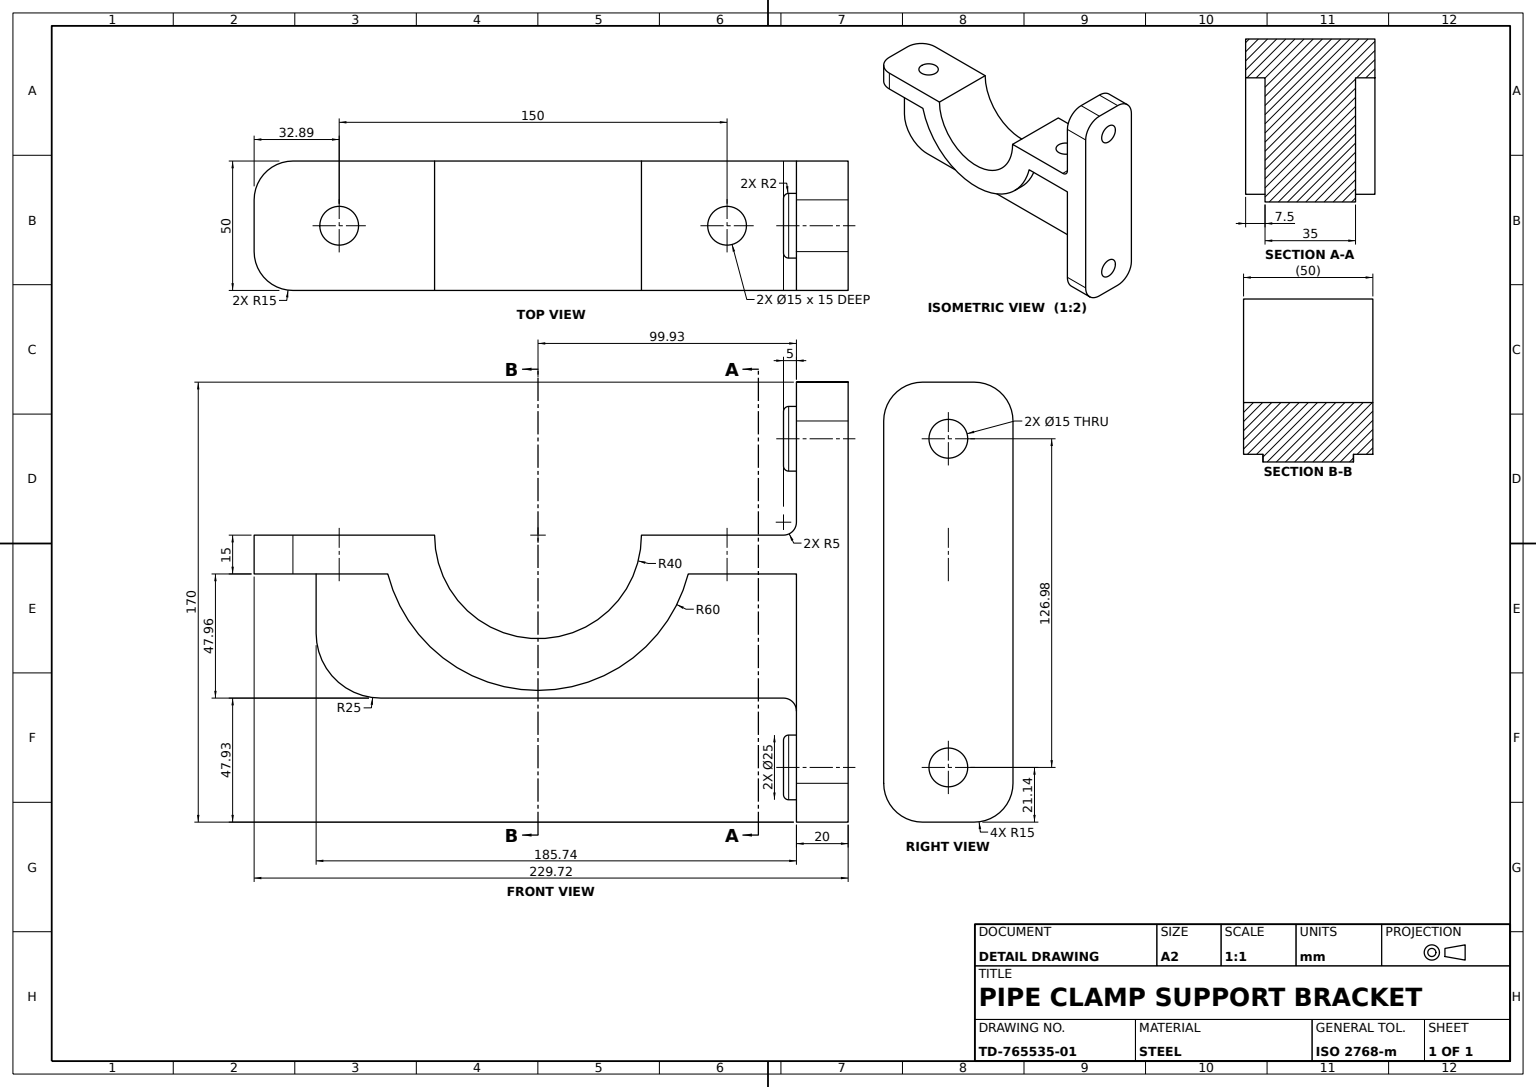
ISO-10303-21;
HEADER;
FILE_DESCRIPTION((''),'2;1');
FILE_NAME('','',(''),(''),'','','');
FILE_SCHEMA(('AUTOMOTIVE_DESIGN'));
ENDSEC;
DATA;
#1=APPLICATION_CONTEXT('');
#2=PRODUCT_CONTEXT('',#1,'mechanical');
#3=PRODUCT('','','',(#2));
#4=PRODUCT_DEFINITION_FORMATION('','',#3);
#5=PRODUCT_DEFINITION_CONTEXT('',#1,'design');
#6=PRODUCT_DEFINITION('','',#4,#5);
#7=PRODUCT_DEFINITION_SHAPE('','',#6);
#8=(LENGTH_UNIT()NAMED_UNIT(*)SI_UNIT(.MILLI.,.METRE.));
#9=(NAMED_UNIT(*)PLANE_ANGLE_UNIT()SI_UNIT($,.RADIAN.));
#10=(NAMED_UNIT(*)SI_UNIT($,.STERADIAN.)SOLID_ANGLE_UNIT());
#11=UNCERTAINTY_MEASURE_WITH_UNIT(LENGTH_MEASURE(1.E-05),#8,'distance_accuracy_value','');
#12=(GEOMETRIC_REPRESENTATION_CONTEXT(3)GLOBAL_UNCERTAINTY_ASSIGNED_CONTEXT((#11))GLOBAL_UNIT_ASSIGNED_CONTEXT((#8,#9,#10))REPRESENTATION_CONTEXT('',''));
#13=CARTESIAN_POINT('',(-17.5,10.889968,205.743047));
#14=VERTEX_POINT('',#13);
#15=CARTESIAN_POINT('',(-17.5,-12.074588,205.743047));
#16=VERTEX_POINT('',#15);
#17=DIRECTION('',(0.,-1.,0.));
#18=VECTOR('',#17,1000.);
#19=LINE('',#13,#18);
#20=EDGE_CURVE('',#14,#16,#19,.T.);
#21=ORIENTED_EDGE('',*,*,#20,.F.);
#22=CARTESIAN_POINT('',(-17.5,10.889968,178.029229));
#23=VERTEX_POINT('',#22);
#24=DIRECTION('',(0.,0.,1.));
#25=VECTOR('',#24,1000.);
#26=LINE('',#22,#25);
#27=EDGE_CURVE('',#23,#14,#26,.T.);
#28=ORIENTED_EDGE('',*,*,#27,.F.);
#29=CARTESIAN_POINT('',(-17.5,10.889968,61.839729));
#30=VERTEX_POINT('',#29);
#31=CARTESIAN_POINT('',(-17.5,25.889968,119.934479));
#32=DIRECTION('',(-1.,0.,0.));
#33=DIRECTION('',(0.,0.,-1.));
#34=AXIS2_PLACEMENT_3D('',#31,#32,#33);
#35=CIRCLE('',#34,60.);
#36=EDGE_CURVE('',#30,#23,#35,.T.);
#37=ORIENTED_EDGE('',*,*,#36,.F.);
#38=CARTESIAN_POINT('',(-17.5,10.889968,20.));
#39=VERTEX_POINT('',#38);
#40=LINE('',#29,#25);
#41=EDGE_CURVE('',#39,#30,#40,.T.);
#42=ORIENTED_EDGE('',*,*,#41,.F.);
#43=CARTESIAN_POINT('',(-17.5,-42.074588,20.));
#44=VERTEX_POINT('',#43);
#45=DIRECTION('',(0.,1.,0.));
#46=VECTOR('',#45,1000.);
#47=LINE('',#38,#46);
#48=EDGE_CURVE('',#44,#39,#47,.T.);
#49=ORIENTED_EDGE('',*,*,#48,.F.);
#50=CARTESIAN_POINT('',(-17.5,-37.074588,25.));
#51=VERTEX_POINT('',#50);
#52=CARTESIAN_POINT('',(-17.5,-42.074588,25.));
#53=DIRECTION('',(1.,0.,0.));
#54=AXIS2_PLACEMENT_3D('',#52,#53,#33);
#55=CIRCLE('',#54,5.);
#56=EDGE_CURVE('',#44,#51,#55,.T.);
#57=ORIENTED_EDGE('',*,*,#56,.T.);
#58=CARTESIAN_POINT('',(-17.5,-37.074588,180.743047));
#59=VERTEX_POINT('',#58);
#60=CARTESIAN_POINT('',(-17.5,-37.074588,205.743047));
#61=VECTOR('',#33,1000.);
#62=LINE('',#60,#61);
#63=EDGE_CURVE('',#59,#51,#62,.T.);
#64=ORIENTED_EDGE('',*,*,#63,.F.);
#65=CARTESIAN_POINT('',(-17.5,-12.074588,180.743047));
#66=AXIS2_PLACEMENT_3D('',#65,#32,#33);
#67=CIRCLE('',#66,25.);
#68=EDGE_CURVE('',#59,#16,#67,.T.);
#69=ORIENTED_EDGE('',*,*,#68,.T.);
#70=EDGE_LOOP('',(#21,#28,#37,#42,#49,#57,#64,#69));
#71=FACE_OUTER_BOUND('',#70,.T.);
#72=AXIS2_PLACEMENT_3D('',#31,#53,#33);
#73=PLANE('',#72);
#74=ADVANCED_FACE('',(#71),#73,.F.);
#75=CARTESIAN_POINT('',(25.,25.889968,79.934479));
#76=VERTEX_POINT('',#75);
#77=CARTESIAN_POINT('',(-25.,25.889968,79.934479));
#78=VERTEX_POINT('',#77);
#79=VECTOR('',#32,1000.);
#80=LINE('',#75,#79);
#81=EDGE_CURVE('',#76,#78,#80,.T.);
#82=ORIENTED_EDGE('',*,*,#81,.F.);
#83=CARTESIAN_POINT('',(25.,25.889968,25.));
#84=VERTEX_POINT('',#83);
#85=LINE('',#75,#61);
#86=EDGE_CURVE('',#76,#84,#85,.T.);
#87=ORIENTED_EDGE('',*,*,#86,.T.);
#88=CARTESIAN_POINT('',(-25.,25.889968,25.));
#89=VERTEX_POINT('',#88);
#90=LINE('',#88,#79);
#91=EDGE_CURVE('',#84,#89,#90,.T.);
#92=ORIENTED_EDGE('',*,*,#91,.T.);
#93=LINE('',#77,#61);
#94=EDGE_CURVE('',#78,#89,#93,.T.);
#95=ORIENTED_EDGE('',*,*,#94,.F.);
#96=EDGE_LOOP('',(#82,#87,#92,#95));
#97=FACE_OUTER_BOUND('',#96,.T.);
#98=CARTESIAN_POINT('',(0.,25.889968,54.322731));
#99=VERTEX_POINT('',#98);
#100=CARTESIAN_POINT('',(0.,25.889968,39.322731));
#101=VERTEX_POINT('',#100);
#102=CARTESIAN_POINT('',(0.,25.889968,46.822731));
#103=AXIS2_PLACEMENT_3D('',#102,#45,#24);
#104=CIRCLE('',#103,7.5);
#105=EDGE_CURVE('',#99,#101,#104,.T.);
#106=ORIENTED_EDGE('',*,*,#105,.F.);
#107=EDGE_CURVE('',#101,#99,#104,.T.);
#108=ORIENTED_EDGE('',*,*,#107,.F.);
#109=EDGE_LOOP('',(#106,#108));
#110=FACE_BOUND('',#109,.T.);
#111=AXIS2_PLACEMENT_3D('',#75,#45,#24);
#112=PLANE('',#111);
#113=ADVANCED_FACE('',(#97,#110),#112,.T.);
#114=CARTESIAN_POINT('',(10.,25.889968,229.717626));
#115=VERTEX_POINT('',#114);
#116=CARTESIAN_POINT('',(25.,25.889968,214.717626));
#117=VERTEX_POINT('',#116);
#118=CARTESIAN_POINT('',(10.,25.889968,214.717626));
#119=AXIS2_PLACEMENT_3D('',#118,#45,#33);
#120=CIRCLE('',#119,15.);
#121=EDGE_CURVE('',#115,#117,#120,.T.);
#122=ORIENTED_EDGE('',*,*,#121,.F.);
#123=CARTESIAN_POINT('',(10.,10.889968,229.717626));
#124=VERTEX_POINT('',#123);
#125=LINE('',#114,#46);
#126=EDGE_CURVE('',#124,#115,#125,.T.);
#127=ORIENTED_EDGE('',*,*,#126,.F.);
#128=CARTESIAN_POINT('',(25.,10.889968,214.717626));
#129=VERTEX_POINT('',#128);
#130=CARTESIAN_POINT('',(10.,10.889968,214.717626));
#131=AXIS2_PLACEMENT_3D('',#130,#17,#33);
#132=CIRCLE('',#131,15.);
#133=EDGE_CURVE('',#129,#124,#132,.T.);
#134=ORIENTED_EDGE('',*,*,#133,.F.);
#135=LINE('',#128,#18);
#136=EDGE_CURVE('',#117,#129,#135,.T.);
#137=ORIENTED_EDGE('',*,*,#136,.F.);
#138=EDGE_LOOP('',(#122,#127,#134,#137));
#139=FACE_OUTER_BOUND('',#138,.T.);
#140=AXIS2_PLACEMENT_3D('',#130,#17,#53);
#141=CYLINDRICAL_SURFACE('',#140,15.);
#142=ADVANCED_FACE('',(#139),#141,.T.);
#143=CARTESIAN_POINT('',(7.5,-63.86192,25.));
#144=VERTEX_POINT('',#143);
#145=CARTESIAN_POINT('',(-7.5,-63.86192,25.));
#146=VERTEX_POINT('',#145);
#147=CARTESIAN_POINT('',(0.,-63.86192,25.));
#148=AXIS2_PLACEMENT_3D('',#147,#24,#53);
#149=CIRCLE('',#148,7.5);
#150=EDGE_CURVE('',#144,#146,#149,.T.);
#151=ORIENTED_EDGE('',*,*,#150,.T.);
#152=CARTESIAN_POINT('',(-7.5,-63.86192,0.));
#153=VERTEX_POINT('',#152);
#154=CARTESIAN_POINT('',(-7.5,-63.86192,-5.));
#155=LINE('',#154,#25);
#156=EDGE_CURVE('',#153,#146,#155,.T.);
#157=ORIENTED_EDGE('',*,*,#156,.F.);
#158=CARTESIAN_POINT('',(7.5,-63.86192,0.));
#159=VERTEX_POINT('',#158);
#160=CARTESIAN_POINT('',(0.,-63.86192,0.));
#161=AXIS2_PLACEMENT_3D('',#160,#24,#53);
#162=CIRCLE('',#161,7.5);
#163=EDGE_CURVE('',#159,#153,#162,.T.);
#164=ORIENTED_EDGE('',*,*,#163,.F.);
#165=CARTESIAN_POINT('',(7.5,-63.86192,-5.));
#166=LINE('',#165,#25);
#167=EDGE_CURVE('',#159,#144,#166,.T.);
#168=ORIENTED_EDGE('',*,*,#167,.T.);
#169=EDGE_LOOP('',(#151,#157,#164,#168));
#170=FACE_OUTER_BOUND('',#169,.T.);
#171=CARTESIAN_POINT('',(0.,-63.86192,-5.));
#172=AXIS2_PLACEMENT_3D('',#171,#24,#53);
#173=CYLINDRICAL_SURFACE('',#172,7.5);
#174=ADVANCED_FACE('',(#170),#173,.F.);
#175=CARTESIAN_POINT('',(7.5,63.122207,0.));
#176=VERTEX_POINT('',#175);
#177=CARTESIAN_POINT('',(-7.5,63.122207,0.));
#178=VERTEX_POINT('',#177);
#179=CARTESIAN_POINT('',(0.,63.122207,0.));
#180=AXIS2_PLACEMENT_3D('',#179,#24,#53);
#181=CIRCLE('',#180,7.5);
#182=EDGE_CURVE('',#176,#178,#181,.T.);
#183=ORIENTED_EDGE('',*,*,#182,.T.);
#184=EDGE_CURVE('',#178,#176,#181,.T.);
#185=ORIENTED_EDGE('',*,*,#184,.T.);
#186=EDGE_LOOP('',(#183,#185));
#187=FACE_BOUND('',#186,.T.);
#188=CARTESIAN_POINT('',(10.,85.,0.));
#189=VERTEX_POINT('',#188);
#190=CARTESIAN_POINT('',(-10.,85.,0.));
#191=VERTEX_POINT('',#190);
#192=CARTESIAN_POINT('',(-25.,85.,0.));
#193=LINE('',#192,#79);
#194=EDGE_CURVE('',#189,#191,#193,.T.);
#195=ORIENTED_EDGE('',*,*,#194,.F.);
#196=CARTESIAN_POINT('',(25.,70.,0.));
#197=VERTEX_POINT('',#196);
#198=CARTESIAN_POINT('',(10.,70.,0.));
#199=AXIS2_PLACEMENT_3D('',#198,#33,#53);
#200=CIRCLE('',#199,15.);
#201=EDGE_CURVE('',#189,#197,#200,.T.);
#202=ORIENTED_EDGE('',*,*,#201,.T.);
#203=CARTESIAN_POINT('',(25.,-70.,0.));
#204=VERTEX_POINT('',#203);
#205=CARTESIAN_POINT('',(25.,85.,0.));
#206=LINE('',#205,#46);
#207=EDGE_CURVE('',#204,#197,#206,.T.);
#208=ORIENTED_EDGE('',*,*,#207,.F.);
#209=CARTESIAN_POINT('',(10.,-85.,0.));
#210=VERTEX_POINT('',#209);
#211=CARTESIAN_POINT('',(10.,-70.,0.));
#212=AXIS2_PLACEMENT_3D('',#211,#33,#53);
#213=CIRCLE('',#212,15.);
#214=EDGE_CURVE('',#204,#210,#213,.T.);
#215=ORIENTED_EDGE('',*,*,#214,.T.);
#216=CARTESIAN_POINT('',(-10.,-85.,0.));
#217=VERTEX_POINT('',#216);
#218=CARTESIAN_POINT('',(-25.,-85.,0.));
#219=VECTOR('',#53,1000.);
#220=LINE('',#218,#219);
#221=EDGE_CURVE('',#217,#210,#220,.T.);
#222=ORIENTED_EDGE('',*,*,#221,.F.);
#223=CARTESIAN_POINT('',(-25.,-70.,0.));
#224=VERTEX_POINT('',#223);
#225=CARTESIAN_POINT('',(-10.,-70.,0.));
#226=AXIS2_PLACEMENT_3D('',#225,#33,#53);
#227=CIRCLE('',#226,15.);
#228=EDGE_CURVE('',#217,#224,#227,.T.);
#229=ORIENTED_EDGE('',*,*,#228,.T.);
#230=CARTESIAN_POINT('',(-25.,70.,0.));
#231=VERTEX_POINT('',#230);
#232=LINE('',#192,#18);
#233=EDGE_CURVE('',#231,#224,#232,.T.);
#234=ORIENTED_EDGE('',*,*,#233,.F.);
#235=CARTESIAN_POINT('',(-10.,70.,0.));
#236=AXIS2_PLACEMENT_3D('',#235,#33,#53);
#237=CIRCLE('',#236,15.);
#238=EDGE_CURVE('',#231,#191,#237,.T.);
#239=ORIENTED_EDGE('',*,*,#238,.T.);
#240=EDGE_LOOP('',(#195,#202,#208,#215,#222,#229,#234,#239));
#241=FACE_OUTER_BOUND('',#240,.T.);
#242=EDGE_CURVE('',#153,#159,#162,.T.);
#243=ORIENTED_EDGE('',*,*,#242,.T.);
#244=ORIENTED_EDGE('',*,*,#163,.T.);
#245=EDGE_LOOP('',(#243,#244));
#246=FACE_BOUND('',#245,.T.);
#247=CARTESIAN_POINT('',(0.,0.,0.));
#248=AXIS2_PLACEMENT_3D('',#247,#24,#53);
#249=PLANE('',#248);
#250=ADVANCED_FACE('',(#187,#241,#246),#249,.F.);
#251=CARTESIAN_POINT('',(-12.5,-63.86192,23.));
#252=VERTEX_POINT('',#251);
#253=CARTESIAN_POINT('',(12.5,-63.86192,23.));
#254=VERTEX_POINT('',#253);
#255=CARTESIAN_POINT('',(0.,-63.86192,23.));
#256=AXIS2_PLACEMENT_3D('',#255,#33,#53);
#257=CIRCLE('',#256,12.5);
#258=EDGE_CURVE('',#252,#254,#257,.T.);
#259=ORIENTED_EDGE('',*,*,#258,.F.);
#260=CARTESIAN_POINT('',(-10.5,-63.86192,25.));
#261=VERTEX_POINT('',#260);
#262=CARTESIAN_POINT('',(-10.5,-63.86192,23.));
#263=AXIS2_PLACEMENT_3D('',#262,#45,#32);
#264=CIRCLE('',#263,2.);
#265=EDGE_CURVE('',#252,#261,#264,.T.);
#266=ORIENTED_EDGE('',*,*,#265,.T.);
#267=CARTESIAN_POINT('',(10.5,-63.86192,25.));
#268=VERTEX_POINT('',#267);
#269=CIRCLE('',#148,10.5);
#270=EDGE_CURVE('',#268,#261,#269,.T.);
#271=ORIENTED_EDGE('',*,*,#270,.F.);
#272=CARTESIAN_POINT('',(10.5,-63.86192,23.));
#273=AXIS2_PLACEMENT_3D('',#272,#17,#33);
#274=CIRCLE('',#273,2.);
#275=EDGE_CURVE('',#254,#268,#274,.T.);
#276=ORIENTED_EDGE('',*,*,#275,.F.);
#277=EDGE_LOOP('',(#259,#266,#271,#276));
#278=FACE_OUTER_BOUND('',#277,.T.);
#279=AXIS2_PLACEMENT_3D('',#255,#24,#53);
#280=TOROIDAL_SURFACE('',#279,10.5,2.);
#281=ADVANCED_FACE('',(#278),#280,.T.);
#282=CARTESIAN_POINT('',(-10.,85.,20.));
#283=VERTEX_POINT('',#282);
#284=CARTESIAN_POINT('',(-25.,70.,20.));
#285=VERTEX_POINT('',#284);
#286=CARTESIAN_POINT('',(-10.,70.,20.));
#287=AXIS2_PLACEMENT_3D('',#286,#24,#53);
#288=CIRCLE('',#287,15.);
#289=EDGE_CURVE('',#283,#285,#288,.T.);
#290=ORIENTED_EDGE('',*,*,#289,.T.);
#291=CARTESIAN_POINT('',(-25.,30.889968,20.));
#292=VERTEX_POINT('',#291);
#293=CARTESIAN_POINT('',(-25.,85.,20.));
#294=LINE('',#293,#18);
#295=EDGE_CURVE('',#285,#292,#294,.T.);
#296=ORIENTED_EDGE('',*,*,#295,.T.);
#297=CARTESIAN_POINT('',(25.,30.889968,20.));
#298=VERTEX_POINT('',#297);
#299=LINE('',#297,#219);
#300=EDGE_CURVE('',#292,#298,#299,.T.);
#301=ORIENTED_EDGE('',*,*,#300,.T.);
#302=CARTESIAN_POINT('',(25.,70.,20.));
#303=VERTEX_POINT('',#302);
#304=CARTESIAN_POINT('',(25.,85.,20.));
#305=LINE('',#304,#46);
#306=EDGE_CURVE('',#298,#303,#305,.T.);
#307=ORIENTED_EDGE('',*,*,#306,.T.);
#308=CARTESIAN_POINT('',(10.,85.,20.));
#309=VERTEX_POINT('',#308);
#310=CARTESIAN_POINT('',(10.,70.,20.));
#311=AXIS2_PLACEMENT_3D('',#310,#24,#53);
#312=CIRCLE('',#311,15.);
#313=EDGE_CURVE('',#303,#309,#312,.T.);
#314=ORIENTED_EDGE('',*,*,#313,.T.);
#315=LINE('',#293,#79);
#316=EDGE_CURVE('',#309,#283,#315,.T.);
#317=ORIENTED_EDGE('',*,*,#316,.T.);
#318=EDGE_LOOP('',(#290,#296,#301,#307,#314,#317));
#319=FACE_OUTER_BOUND('',#318,.T.);
#320=CARTESIAN_POINT('',(12.5,63.122207,20.));
#321=VERTEX_POINT('',#320);
#322=CARTESIAN_POINT('',(-12.5,63.122207,20.));
#323=VERTEX_POINT('',#322);
#324=CARTESIAN_POINT('',(0.,63.122207,20.));
#325=AXIS2_PLACEMENT_3D('',#324,#24,#53);
#326=CIRCLE('',#325,12.5);
#327=EDGE_CURVE('',#321,#323,#326,.T.);
#328=ORIENTED_EDGE('',*,*,#327,.F.);
#329=EDGE_CURVE('',#323,#321,#326,.T.);
#330=ORIENTED_EDGE('',*,*,#329,.F.);
#331=EDGE_LOOP('',(#328,#330));
#332=FACE_BOUND('',#331,.T.);
#333=CARTESIAN_POINT('',(0.,0.,20.));
#334=AXIS2_PLACEMENT_3D('',#333,#24,#53);
#335=PLANE('',#334);
#336=ADVANCED_FACE('',(#319,#332),#335,.T.);
#337=LINE('',#302,#25);
#338=EDGE_CURVE('',#197,#303,#337,.T.);
#339=ORIENTED_EDGE('',*,*,#338,.F.);
#340=ORIENTED_EDGE('',*,*,#201,.F.);
#341=LINE('',#308,#61);
#342=EDGE_CURVE('',#309,#189,#341,.T.);
#343=ORIENTED_EDGE('',*,*,#342,.F.);
#344=ORIENTED_EDGE('',*,*,#313,.F.);
#345=EDGE_LOOP('',(#339,#340,#343,#344));
#346=FACE_OUTER_BOUND('',#345,.T.);
#347=AXIS2_PLACEMENT_3D('',#310,#33,#32);
#348=CYLINDRICAL_SURFACE('',#347,15.);
#349=ADVANCED_FACE('',(#346),#348,.T.);
#350=CARTESIAN_POINT('',(-25.,10.889968,178.029229));
#351=VERTEX_POINT('',#350);
#352=CARTESIAN_POINT('',(25.,10.889968,178.029229));
#353=LINE('',#352,#79);
#354=EDGE_CURVE('',#23,#351,#353,.T.);
#355=ORIENTED_EDGE('',*,*,#354,.T.);
#356=CARTESIAN_POINT('',(-25.,10.889968,61.839729));
#357=VERTEX_POINT('',#356);
#358=CARTESIAN_POINT('',(-25.,25.889968,119.934479));
#359=AXIS2_PLACEMENT_3D('',#358,#53,#33);
#360=CIRCLE('',#359,60.);
#361=EDGE_CURVE('',#351,#357,#360,.T.);
#362=ORIENTED_EDGE('',*,*,#361,.T.);
#363=CARTESIAN_POINT('',(25.,10.889968,61.839729));
#364=LINE('',#363,#79);
#365=EDGE_CURVE('',#30,#357,#364,.T.);
#366=ORIENTED_EDGE('',*,*,#365,.F.);
#367=ORIENTED_EDGE('',*,*,#36,.T.);
#368=EDGE_LOOP('',(#355,#362,#366,#367));
#369=FACE_OUTER_BOUND('',#368,.T.);
#370=CARTESIAN_POINT('',(25.,25.889968,119.934479));
#371=AXIS2_PLACEMENT_3D('',#370,#32,#24);
#372=CYLINDRICAL_SURFACE('',#371,60.);
#373=ADVANCED_FACE('',(#369),#372,.T.);
#374=CARTESIAN_POINT('',(-25.,-70.,20.));
#375=VERTEX_POINT('',#374);
#376=CARTESIAN_POINT('',(-10.,-85.,20.));
#377=VERTEX_POINT('',#376);
#378=CARTESIAN_POINT('',(-10.,-70.,20.));
#379=AXIS2_PLACEMENT_3D('',#378,#24,#53);
#380=CIRCLE('',#379,15.);
#381=EDGE_CURVE('',#375,#377,#380,.T.);
#382=ORIENTED_EDGE('',*,*,#381,.F.);
#383=LINE('',#374,#25);
#384=EDGE_CURVE('',#224,#375,#383,.T.);
#385=ORIENTED_EDGE('',*,*,#384,.F.);
#386=ORIENTED_EDGE('',*,*,#228,.F.);
#387=LINE('',#376,#61);
#388=EDGE_CURVE('',#377,#217,#387,.T.);
#389=ORIENTED_EDGE('',*,*,#388,.F.);
#390=EDGE_LOOP('',(#382,#385,#386,#389));
#391=FACE_OUTER_BOUND('',#390,.T.);
#392=AXIS2_PLACEMENT_3D('',#378,#33,#32);
#393=CYLINDRICAL_SURFACE('',#392,15.);
#394=ADVANCED_FACE('',(#391),#393,.T.);
#395=ORIENTED_EDGE('',*,*,#56,.F.);
#396=CARTESIAN_POINT('',(17.5,-42.074588,20.));
#397=VERTEX_POINT('',#396);
#398=CARTESIAN_POINT('',(0.,-42.074588,20.));
#399=LINE('',#398,#79);
#400=EDGE_CURVE('',#397,#44,#399,.T.);
#401=ORIENTED_EDGE('',*,*,#400,.F.);
#402=CARTESIAN_POINT('',(17.5,-37.074588,25.));
#403=VERTEX_POINT('',#402);
#404=CARTESIAN_POINT('',(17.5,-42.074588,25.));
#405=AXIS2_PLACEMENT_3D('',#404,#32,#33);
#406=CIRCLE('',#405,5.);
#407=EDGE_CURVE('',#403,#397,#406,.T.);
#408=ORIENTED_EDGE('',*,*,#407,.F.);
#409=LINE('',#402,#219);
#410=EDGE_CURVE('',#51,#403,#409,.T.);
#411=ORIENTED_EDGE('',*,*,#410,.F.);
#412=EDGE_LOOP('',(#395,#401,#408,#411));
#413=FACE_OUTER_BOUND('',#412,.T.);
#414=CARTESIAN_POINT('',(0.,-42.074588,25.));
#415=AXIS2_PLACEMENT_3D('',#414,#32,#24);
#416=CYLINDRICAL_SURFACE('',#415,5.);
#417=ADVANCED_FACE('',(#413),#416,.F.);
#418=CARTESIAN_POINT('',(0.,10.889968,204.322731));
#419=VERTEX_POINT('',#418);
#420=CARTESIAN_POINT('',(0.,25.889968,204.322731));
#421=VERTEX_POINT('',#420);
#422=CARTESIAN_POINT('',(0.,0.889968,204.322731));
#423=LINE('',#422,#46);
#424=EDGE_CURVE('',#419,#421,#423,.T.);
#425=ORIENTED_EDGE('',*,*,#424,.T.);
#426=CARTESIAN_POINT('',(0.,25.889968,189.322731));
#427=VERTEX_POINT('',#426);
#428=CARTESIAN_POINT('',(0.,25.889968,196.822731));
#429=AXIS2_PLACEMENT_3D('',#428,#17,#33);
#430=CIRCLE('',#429,7.5);
#431=EDGE_CURVE('',#427,#421,#430,.T.);
#432=ORIENTED_EDGE('',*,*,#431,.F.);
#433=CARTESIAN_POINT('',(0.,10.889968,189.322731));
#434=VERTEX_POINT('',#433);
#435=CARTESIAN_POINT('',(0.,0.889968,189.322731));
#436=LINE('',#435,#46);
#437=EDGE_CURVE('',#434,#427,#436,.T.);
#438=ORIENTED_EDGE('',*,*,#437,.F.);
#439=CARTESIAN_POINT('',(0.,10.889968,196.822731));
#440=AXIS2_PLACEMENT_3D('',#439,#45,#33);
#441=CIRCLE('',#440,7.5);
#442=EDGE_CURVE('',#419,#434,#441,.T.);
#443=ORIENTED_EDGE('',*,*,#442,.F.);
#444=EDGE_LOOP('',(#425,#432,#438,#443));
#445=FACE_OUTER_BOUND('',#444,.T.);
#446=CARTESIAN_POINT('',(0.,0.889968,196.822731));
#447=AXIS2_PLACEMENT_3D('',#446,#45,#24);
#448=CYLINDRICAL_SURFACE('',#447,7.5);
#449=ADVANCED_FACE('',(#445),#448,.F.);
#450=CARTESIAN_POINT('',(-10.,25.889968,229.717626));
#451=VERTEX_POINT('',#450);
#452=CARTESIAN_POINT('',(25.,25.889968,229.717626));
#453=LINE('',#452,#79);
#454=EDGE_CURVE('',#115,#451,#453,.T.);
#455=ORIENTED_EDGE('',*,*,#454,.T.);
#456=CARTESIAN_POINT('',(-10.,10.889968,229.717626));
#457=VERTEX_POINT('',#456);
#458=LINE('',#456,#18);
#459=EDGE_CURVE('',#451,#457,#458,.T.);
#460=ORIENTED_EDGE('',*,*,#459,.T.);
#461=CARTESIAN_POINT('',(25.,10.889968,229.717626));
#462=LINE('',#461,#79);
#463=EDGE_CURVE('',#124,#457,#462,.T.);
#464=ORIENTED_EDGE('',*,*,#463,.F.);
#465=ORIENTED_EDGE('',*,*,#126,.T.);
#466=EDGE_LOOP('',(#455,#460,#464,#465));
#467=FACE_OUTER_BOUND('',#466,.T.);
#468=AXIS2_PLACEMENT_3D('',#461,#24,#53);
#469=PLANE('',#468);
#470=ADVANCED_FACE('',(#467),#469,.T.);
#471=EDGE_CURVE('',#261,#268,#269,.T.);
#472=ORIENTED_EDGE('',*,*,#471,.F.);
#473=ORIENTED_EDGE('',*,*,#265,.F.);
#474=EDGE_CURVE('',#254,#252,#257,.T.);
#475=ORIENTED_EDGE('',*,*,#474,.F.);
#476=ORIENTED_EDGE('',*,*,#275,.T.);
#477=EDGE_LOOP('',(#472,#473,#475,#476));
#478=FACE_OUTER_BOUND('',#477,.T.);
#479=ADVANCED_FACE('',(#478),#280,.T.);
#480=ORIENTED_EDGE('',*,*,#342,.T.);
#481=ORIENTED_EDGE('',*,*,#194,.T.);
#482=LINE('',#282,#25);
#483=EDGE_CURVE('',#191,#283,#482,.T.);
#484=ORIENTED_EDGE('',*,*,#483,.T.);
#485=ORIENTED_EDGE('',*,*,#316,.F.);
#486=EDGE_LOOP('',(#480,#481,#484,#485));
#487=FACE_OUTER_BOUND('',#486,.T.);
#488=AXIS2_PLACEMENT_3D('',#293,#17,#33);
#489=PLANE('',#488);
#490=ADVANCED_FACE('',(#487),#489,.F.);
#491=VERTEX_POINT('',#352);
#492=VERTEX_POINT('',#363);
#493=AXIS2_PLACEMENT_3D('',#370,#53,#33);
#494=CIRCLE('',#493,60.);
#495=EDGE_CURVE('',#491,#492,#494,.T.);
#496=ORIENTED_EDGE('',*,*,#495,.F.);
#497=CARTESIAN_POINT('',(17.5,10.889968,178.029229));
#498=VERTEX_POINT('',#497);
#499=EDGE_CURVE('',#491,#498,#353,.T.);
#500=ORIENTED_EDGE('',*,*,#499,.T.);
#501=CARTESIAN_POINT('',(17.5,10.889968,61.839729));
#502=VERTEX_POINT('',#501);
#503=CARTESIAN_POINT('',(17.5,25.889968,119.934479));
#504=AXIS2_PLACEMENT_3D('',#503,#32,#33);
#505=CIRCLE('',#504,60.);
#506=EDGE_CURVE('',#502,#498,#505,.T.);
#507=ORIENTED_EDGE('',*,*,#506,.F.);
#508=EDGE_CURVE('',#492,#502,#364,.T.);
#509=ORIENTED_EDGE('',*,*,#508,.F.);
#510=EDGE_LOOP('',(#496,#500,#507,#509));
#511=FACE_OUTER_BOUND('',#510,.T.);
#512=ADVANCED_FACE('',(#511),#372,.T.);
#513=CARTESIAN_POINT('',(25.,30.889968,25.));
#514=AXIS2_PLACEMENT_3D('',#513,#32,#17);
#515=CIRCLE('',#514,5.);
#516=EDGE_CURVE('',#298,#84,#515,.T.);
#517=ORIENTED_EDGE('',*,*,#516,.F.);
#518=ORIENTED_EDGE('',*,*,#300,.F.);
#519=CARTESIAN_POINT('',(-25.,30.889968,25.));
#520=AXIS2_PLACEMENT_3D('',#519,#53,#45);
#521=CIRCLE('',#520,5.);
#522=EDGE_CURVE('',#89,#292,#521,.T.);
#523=ORIENTED_EDGE('',*,*,#522,.F.);
#524=ORIENTED_EDGE('',*,*,#91,.F.);
#525=EDGE_LOOP('',(#517,#518,#523,#524));
#526=FACE_OUTER_BOUND('',#525,.T.);
#527=AXIS2_PLACEMENT_3D('',#513,#53,#33);
#528=CYLINDRICAL_SURFACE('',#527,5.);
#529=ADVANCED_FACE('',(#526),#528,.F.);
#530=CARTESIAN_POINT('',(0.,10.889968,54.322731));
#531=VERTEX_POINT('',#530);
#532=CARTESIAN_POINT('',(0.,0.889968,54.322731));
#533=LINE('',#532,#46);
#534=EDGE_CURVE('',#531,#99,#533,.T.);
#535=ORIENTED_EDGE('',*,*,#534,.F.);
#536=CARTESIAN_POINT('',(0.,10.889968,39.322731));
#537=VERTEX_POINT('',#536);
#538=CARTESIAN_POINT('',(0.,10.889968,46.822731));
#539=AXIS2_PLACEMENT_3D('',#538,#45,#24);
#540=CIRCLE('',#539,7.5);
#541=EDGE_CURVE('',#537,#531,#540,.T.);
#542=ORIENTED_EDGE('',*,*,#541,.F.);
#543=CARTESIAN_POINT('',(0.,0.889968,39.322731));
#544=LINE('',#543,#46);
#545=EDGE_CURVE('',#537,#101,#544,.T.);
#546=ORIENTED_EDGE('',*,*,#545,.T.);
#547=ORIENTED_EDGE('',*,*,#107,.T.);
#548=EDGE_LOOP('',(#535,#542,#546,#547));
#549=FACE_OUTER_BOUND('',#548,.T.);
#550=CARTESIAN_POINT('',(0.,0.889968,46.822731));
#551=AXIS2_PLACEMENT_3D('',#550,#45,#24);
#552=CYLINDRICAL_SURFACE('',#551,7.5);
#553=ADVANCED_FACE('',(#549),#552,.F.);
#554=ORIENTED_EDGE('',*,*,#516,.T.);
#555=ORIENTED_EDGE('',*,*,#86,.F.);
#556=CARTESIAN_POINT('',(25.,25.889968,159.934479));
#557=VERTEX_POINT('',#556);
#558=CIRCLE('',#493,40.);
#559=EDGE_CURVE('',#557,#76,#558,.T.);
#560=ORIENTED_EDGE('',*,*,#559,.F.);
#561=CARTESIAN_POINT('',(25.,25.889968,179.934479));
#562=LINE('',#561,#25);
#563=EDGE_CURVE('',#557,#117,#562,.T.);
#564=ORIENTED_EDGE('',*,*,#563,.T.);
#565=ORIENTED_EDGE('',*,*,#136,.T.);
#566=LINE('',#352,#25);
#567=EDGE_CURVE('',#491,#129,#566,.T.);
#568=ORIENTED_EDGE('',*,*,#567,.F.);
#569=ORIENTED_EDGE('',*,*,#495,.T.);
#570=CARTESIAN_POINT('',(25.,10.889968,20.));
#571=VERTEX_POINT('',#570);
#572=LINE('',#363,#61);
#573=EDGE_CURVE('',#492,#571,#572,.T.);
#574=ORIENTED_EDGE('',*,*,#573,.T.);
#575=CARTESIAN_POINT('',(25.,-70.,20.));
#576=VERTEX_POINT('',#575);
#577=EDGE_CURVE('',#576,#571,#305,.T.);
#578=ORIENTED_EDGE('',*,*,#577,.F.);
#579=LINE('',#575,#61);
#580=EDGE_CURVE('',#576,#204,#579,.T.);
#581=ORIENTED_EDGE('',*,*,#580,.T.);
#582=ORIENTED_EDGE('',*,*,#207,.T.);
#583=ORIENTED_EDGE('',*,*,#338,.T.);
#584=ORIENTED_EDGE('',*,*,#306,.F.);
#585=EDGE_LOOP('',(#554,#555,#560,#564,#565,#568,#569,#574,#578,#581,#582,#583,#584));
#586=FACE_OUTER_BOUND('',#585,.T.);
#587=AXIS2_PLACEMENT_3D('',#304,#32,#17);
#588=PLANE('',#587);
#589=ADVANCED_FACE('',(#586),#588,.F.);
#590=CARTESIAN_POINT('',(10.,-85.,20.));
#591=VERTEX_POINT('',#590);
#592=LINE('',#590,#25);
#593=EDGE_CURVE('',#210,#591,#592,.T.);
#594=ORIENTED_EDGE('',*,*,#593,.T.);
#595=CARTESIAN_POINT('',(-25.,-85.,20.));
#596=LINE('',#595,#219);
#597=EDGE_CURVE('',#377,#591,#596,.T.);
#598=ORIENTED_EDGE('',*,*,#597,.F.);
#599=ORIENTED_EDGE('',*,*,#388,.T.);
#600=ORIENTED_EDGE('',*,*,#221,.T.);
#601=EDGE_LOOP('',(#594,#598,#599,#600));
#602=FACE_OUTER_BOUND('',#601,.T.);
#603=AXIS2_PLACEMENT_3D('',#595,#45,#24);
#604=PLANE('',#603);
#605=ADVANCED_FACE('',(#602),#604,.F.);
#606=CARTESIAN_POINT('',(-12.5,-63.86192,20.));
#607=VERTEX_POINT('',#606);
#608=CARTESIAN_POINT('',(-12.5,-63.86192,25.));
#609=LINE('',#608,#61);
#610=EDGE_CURVE('',#252,#607,#609,.T.);
#611=ORIENTED_EDGE('',*,*,#610,.F.);
#612=ORIENTED_EDGE('',*,*,#258,.T.);
#613=CARTESIAN_POINT('',(12.5,-63.86192,20.));
#614=VERTEX_POINT('',#613);
#615=CARTESIAN_POINT('',(12.5,-63.86192,25.));
#616=LINE('',#615,#61);
#617=EDGE_CURVE('',#254,#614,#616,.T.);
#618=ORIENTED_EDGE('',*,*,#617,.T.);
#619=CARTESIAN_POINT('',(0.,-63.86192,20.));
#620=AXIS2_PLACEMENT_3D('',#619,#24,#53);
#621=CIRCLE('',#620,12.5);
#622=EDGE_CURVE('',#614,#607,#621,.T.);
#623=ORIENTED_EDGE('',*,*,#622,.T.);
#624=EDGE_LOOP('',(#611,#612,#618,#623));
#625=FACE_OUTER_BOUND('',#624,.T.);
#626=AXIS2_PLACEMENT_3D('',#147,#33,#32);
#627=CYLINDRICAL_SURFACE('',#626,12.5);
#628=ADVANCED_FACE('',(#625),#627,.T.);
#629=CARTESIAN_POINT('',(-7.5,63.122207,25.));
#630=VERTEX_POINT('',#629);
#631=CARTESIAN_POINT('',(7.5,63.122207,25.));
#632=VERTEX_POINT('',#631);
#633=CARTESIAN_POINT('',(0.,63.122207,25.));
#634=AXIS2_PLACEMENT_3D('',#633,#24,#53);
#635=CIRCLE('',#634,7.5);
#636=EDGE_CURVE('',#630,#632,#635,.T.);
#637=ORIENTED_EDGE('',*,*,#636,.F.);
#638=EDGE_CURVE('',#632,#630,#635,.T.);
#639=ORIENTED_EDGE('',*,*,#638,.F.);
#640=EDGE_LOOP('',(#637,#639));
#641=FACE_BOUND('',#640,.T.);
#642=CARTESIAN_POINT('',(10.5,63.122207,25.));
#643=VERTEX_POINT('',#642);
#644=CARTESIAN_POINT('',(-10.5,63.122207,25.));
#645=VERTEX_POINT('',#644);
#646=CIRCLE('',#634,10.5);
#647=EDGE_CURVE('',#643,#645,#646,.T.);
#648=ORIENTED_EDGE('',*,*,#647,.T.);
#649=EDGE_CURVE('',#645,#643,#646,.T.);
#650=ORIENTED_EDGE('',*,*,#649,.T.);
#651=EDGE_LOOP('',(#648,#650));
#652=FACE_OUTER_BOUND('',#651,.T.);
#653=PLANE('',#634);
#654=ADVANCED_FACE('',(#641,#652),#653,.T.);
#655=EDGE_CURVE('',#531,#537,#540,.T.);
#656=ORIENTED_EDGE('',*,*,#655,.F.);
#657=ORIENTED_EDGE('',*,*,#534,.T.);
#658=ORIENTED_EDGE('',*,*,#105,.T.);
#659=ORIENTED_EDGE('',*,*,#545,.F.);
#660=EDGE_LOOP('',(#656,#657,#658,#659));
#661=FACE_OUTER_BOUND('',#660,.T.);
#662=ADVANCED_FACE('',(#661),#552,.F.);
#663=CARTESIAN_POINT('',(-25.,10.889968,214.717626));
#664=VERTEX_POINT('',#663);
#665=CARTESIAN_POINT('',(-10.,10.889968,214.717626));
#666=AXIS2_PLACEMENT_3D('',#665,#17,#33);
#667=CIRCLE('',#666,15.);
#668=EDGE_CURVE('',#457,#664,#667,.T.);
#669=ORIENTED_EDGE('',*,*,#668,.F.);
#670=ORIENTED_EDGE('',*,*,#459,.F.);
#671=CARTESIAN_POINT('',(-25.,25.889968,214.717626));
#672=VERTEX_POINT('',#671);
#673=CARTESIAN_POINT('',(-10.,25.889968,214.717626));
#674=AXIS2_PLACEMENT_3D('',#673,#45,#33);
#675=CIRCLE('',#674,15.);
#676=EDGE_CURVE('',#672,#451,#675,.T.);
#677=ORIENTED_EDGE('',*,*,#676,.F.);
#678=LINE('',#671,#46);
#679=EDGE_CURVE('',#664,#672,#678,.T.);
#680=ORIENTED_EDGE('',*,*,#679,.F.);
#681=EDGE_LOOP('',(#669,#670,#677,#680));
#682=FACE_OUTER_BOUND('',#681,.T.);
#683=CARTESIAN_POINT('',(-10.,85.,214.717626));
#684=AXIS2_PLACEMENT_3D('',#683,#17,#53);
#685=CYLINDRICAL_SURFACE('',#684,15.);
#686=ADVANCED_FACE('',(#682),#685,.T.);
#687=LINE('',#350,#25);
#688=EDGE_CURVE('',#351,#664,#687,.T.);
#689=ORIENTED_EDGE('',*,*,#688,.F.);
#690=ORIENTED_EDGE('',*,*,#354,.F.);
#691=ORIENTED_EDGE('',*,*,#27,.T.);
#692=CARTESIAN_POINT('',(17.5,10.889968,205.743047));
#693=VERTEX_POINT('',#692);
#694=LINE('',#692,#79);
#695=EDGE_CURVE('',#693,#14,#694,.T.);
#696=ORIENTED_EDGE('',*,*,#695,.F.);
#697=LINE('',#497,#25);
#698=EDGE_CURVE('',#498,#693,#697,.T.);
#699=ORIENTED_EDGE('',*,*,#698,.F.);
#700=ORIENTED_EDGE('',*,*,#499,.F.);
#701=ORIENTED_EDGE('',*,*,#567,.T.);
#702=ORIENTED_EDGE('',*,*,#133,.T.);
#703=ORIENTED_EDGE('',*,*,#463,.T.);
#704=ORIENTED_EDGE('',*,*,#668,.T.);
#705=EDGE_LOOP('',(#689,#690,#691,#696,#699,#700,#701,#702,#703,#704));
#706=FACE_OUTER_BOUND('',#705,.T.);
#707=AXIS2_PLACEMENT_3D('',#352,#17,#33);
#708=PLANE('',#707);
#709=ADVANCED_FACE('',(#706),#708,.T.);
#710=ORIENTED_EDGE('',*,*,#182,.F.);
#711=CARTESIAN_POINT('',(7.5,63.122207,-5.));
#712=LINE('',#711,#25);
#713=EDGE_CURVE('',#176,#632,#712,.T.);
#714=ORIENTED_EDGE('',*,*,#713,.T.);
#715=ORIENTED_EDGE('',*,*,#638,.T.);
#716=CARTESIAN_POINT('',(-7.5,63.122207,-5.));
#717=LINE('',#716,#25);
#718=EDGE_CURVE('',#178,#630,#717,.T.);
#719=ORIENTED_EDGE('',*,*,#718,.F.);
#720=EDGE_LOOP('',(#710,#714,#715,#719));
#721=FACE_OUTER_BOUND('',#720,.T.);
#722=CARTESIAN_POINT('',(0.,63.122207,-5.));
#723=AXIS2_PLACEMENT_3D('',#722,#24,#53);
#724=CYLINDRICAL_SURFACE('',#723,7.5);
#725=ADVANCED_FACE('',(#721),#724,.F.);
#726=CARTESIAN_POINT('',(12.5,63.122207,23.));
#727=VERTEX_POINT('',#726);
#728=CARTESIAN_POINT('',(12.5,63.122207,25.));
#729=LINE('',#728,#61);
#730=EDGE_CURVE('',#727,#321,#729,.T.);
#731=ORIENTED_EDGE('',*,*,#730,.T.);
#732=ORIENTED_EDGE('',*,*,#327,.T.);
#733=CARTESIAN_POINT('',(-12.5,63.122207,23.));
#734=VERTEX_POINT('',#733);
#735=CARTESIAN_POINT('',(-12.5,63.122207,25.));
#736=LINE('',#735,#61);
#737=EDGE_CURVE('',#734,#323,#736,.T.);
#738=ORIENTED_EDGE('',*,*,#737,.F.);
#739=CARTESIAN_POINT('',(0.,63.122207,23.));
#740=AXIS2_PLACEMENT_3D('',#739,#33,#53);
#741=CIRCLE('',#740,12.5);
#742=EDGE_CURVE('',#734,#727,#741,.T.);
#743=ORIENTED_EDGE('',*,*,#742,.T.);
#744=EDGE_LOOP('',(#731,#732,#738,#743));
#745=FACE_OUTER_BOUND('',#744,.T.);
#746=AXIS2_PLACEMENT_3D('',#633,#33,#32);
#747=CYLINDRICAL_SURFACE('',#746,12.5);
#748=ADVANCED_FACE('',(#745),#747,.T.);
#749=ORIENTED_EDGE('',*,*,#410,.T.);
#750=CARTESIAN_POINT('',(17.5,-37.074588,180.743047));
#751=VERTEX_POINT('',#750);
#752=CARTESIAN_POINT('',(17.5,-37.074588,205.743047));
#753=LINE('',#752,#61);
#754=EDGE_CURVE('',#751,#403,#753,.T.);
#755=ORIENTED_EDGE('',*,*,#754,.F.);
#756=LINE('',#750,#79);
#757=EDGE_CURVE('',#751,#59,#756,.T.);
#758=ORIENTED_EDGE('',*,*,#757,.T.);
#759=ORIENTED_EDGE('',*,*,#63,.T.);
#760=EDGE_LOOP('',(#749,#755,#758,#759));
#761=FACE_OUTER_BOUND('',#760,.T.);
#762=AXIS2_PLACEMENT_3D('',#752,#45,#24);
#763=PLANE('',#762);
#764=ADVANCED_FACE('',(#761),#763,.F.);
#765=CARTESIAN_POINT('',(17.5,-12.074588,205.743047));
#766=VERTEX_POINT('',#765);
#767=LINE('',#692,#18);
#768=EDGE_CURVE('',#693,#766,#767,.T.);
#769=ORIENTED_EDGE('',*,*,#768,.F.);
#770=ORIENTED_EDGE('',*,*,#695,.T.);
#771=ORIENTED_EDGE('',*,*,#20,.T.);
#772=LINE('',#765,#219);
#773=EDGE_CURVE('',#16,#766,#772,.T.);
#774=ORIENTED_EDGE('',*,*,#773,.T.);
#775=EDGE_LOOP('',(#769,#770,#771,#774));
#776=FACE_OUTER_BOUND('',#775,.T.);
#777=AXIS2_PLACEMENT_3D('',#692,#33,#32);
#778=PLANE('',#777);
#779=ADVANCED_FACE('',(#776),#778,.F.);
#780=ORIENTED_EDGE('',*,*,#718,.T.);
#781=ORIENTED_EDGE('',*,*,#636,.T.);
#782=ORIENTED_EDGE('',*,*,#713,.F.);
#783=ORIENTED_EDGE('',*,*,#184,.F.);
#784=EDGE_LOOP('',(#780,#781,#782,#783));
#785=FACE_OUTER_BOUND('',#784,.T.);
#786=ADVANCED_FACE('',(#785),#724,.F.);
#787=ORIENTED_EDGE('',*,*,#238,.F.);
#788=LINE('',#284,#61);
#789=EDGE_CURVE('',#285,#231,#788,.T.);
#790=ORIENTED_EDGE('',*,*,#789,.F.);
#791=ORIENTED_EDGE('',*,*,#289,.F.);
#792=ORIENTED_EDGE('',*,*,#483,.F.);
#793=EDGE_LOOP('',(#787,#790,#791,#792));
#794=FACE_OUTER_BOUND('',#793,.T.);
#795=AXIS2_PLACEMENT_3D('',#286,#33,#32);
#796=CYLINDRICAL_SURFACE('',#795,15.);
#797=ADVANCED_FACE('',(#794),#796,.T.);
#798=ORIENTED_EDGE('',*,*,#508,.T.);
#799=CARTESIAN_POINT('',(17.5,10.889968,20.));
#800=VERTEX_POINT('',#799);
#801=LINE('',#501,#25);
#802=EDGE_CURVE('',#800,#502,#801,.T.);
#803=ORIENTED_EDGE('',*,*,#802,.F.);
#804=LINE('',#570,#79);
#805=EDGE_CURVE('',#571,#800,#804,.T.);
#806=ORIENTED_EDGE('',*,*,#805,.F.);
#807=ORIENTED_EDGE('',*,*,#573,.F.);
#808=EDGE_LOOP('',(#798,#803,#806,#807));
#809=FACE_OUTER_BOUND('',#808,.T.);
#810=AXIS2_PLACEMENT_3D('',#363,#45,#24);
#811=PLANE('',#810);
#812=ADVANCED_FACE('',(#809),#811,.F.);
#813=EDGE_CURVE('',#434,#419,#441,.T.);
#814=ORIENTED_EDGE('',*,*,#813,.F.);
#815=ORIENTED_EDGE('',*,*,#437,.T.);
#816=EDGE_CURVE('',#421,#427,#430,.T.);
#817=ORIENTED_EDGE('',*,*,#816,.F.);
#818=ORIENTED_EDGE('',*,*,#424,.F.);
#819=EDGE_LOOP('',(#814,#815,#817,#818));
#820=FACE_OUTER_BOUND('',#819,.T.);
#821=ADVANCED_FACE('',(#820),#448,.F.);
#822=CARTESIAN_POINT('',(-25.,25.889968,159.934479));
#823=VERTEX_POINT('',#822);
#824=LINE('',#556,#79);
#825=EDGE_CURVE('',#557,#823,#824,.T.);
#826=ORIENTED_EDGE('',*,*,#825,.F.);
#827=ORIENTED_EDGE('',*,*,#559,.T.);
#828=ORIENTED_EDGE('',*,*,#81,.T.);
#829=CIRCLE('',#359,40.);
#830=EDGE_CURVE('',#823,#78,#829,.T.);
#831=ORIENTED_EDGE('',*,*,#830,.F.);
#832=EDGE_LOOP('',(#826,#827,#828,#831));
#833=FACE_OUTER_BOUND('',#832,.T.);
#834=CYLINDRICAL_SURFACE('',#371,40.);
#835=ADVANCED_FACE('',(#833),#834,.F.);
#836=ORIENTED_EDGE('',*,*,#94,.T.);
#837=ORIENTED_EDGE('',*,*,#522,.T.);
#838=ORIENTED_EDGE('',*,*,#295,.F.);
#839=ORIENTED_EDGE('',*,*,#789,.T.);
#840=ORIENTED_EDGE('',*,*,#233,.T.);
#841=ORIENTED_EDGE('',*,*,#384,.T.);
#842=CARTESIAN_POINT('',(-25.,10.889968,20.));
#843=VERTEX_POINT('',#842);
#844=EDGE_CURVE('',#843,#375,#294,.T.);
#845=ORIENTED_EDGE('',*,*,#844,.F.);
#846=LINE('',#356,#61);
#847=EDGE_CURVE('',#357,#843,#846,.T.);
#848=ORIENTED_EDGE('',*,*,#847,.F.);
#849=ORIENTED_EDGE('',*,*,#361,.F.);
#850=ORIENTED_EDGE('',*,*,#688,.T.);
#851=ORIENTED_EDGE('',*,*,#679,.T.);
#852=LINE('',#822,#25);
#853=EDGE_CURVE('',#823,#672,#852,.T.);
#854=ORIENTED_EDGE('',*,*,#853,.F.);
#855=ORIENTED_EDGE('',*,*,#830,.T.);
#856=EDGE_LOOP('',(#836,#837,#838,#839,#840,#841,#845,#848,#849,#850,#851,#854,#855));
#857=FACE_OUTER_BOUND('',#856,.T.);
#858=AXIS2_PLACEMENT_3D('',#293,#53,#45);
#859=PLANE('',#858);
#860=ADVANCED_FACE('',(#857),#859,.F.);
#861=CARTESIAN_POINT('',(-10.5,63.122207,23.));
#862=AXIS2_PLACEMENT_3D('',#861,#45,#32);
#863=CIRCLE('',#862,2.);
#864=EDGE_CURVE('',#734,#645,#863,.T.);
#865=ORIENTED_EDGE('',*,*,#864,.T.);
#866=ORIENTED_EDGE('',*,*,#647,.F.);
#867=CARTESIAN_POINT('',(10.5,63.122207,23.));
#868=AXIS2_PLACEMENT_3D('',#867,#17,#33);
#869=CIRCLE('',#868,2.);
#870=EDGE_CURVE('',#727,#643,#869,.T.);
#871=ORIENTED_EDGE('',*,*,#870,.F.);
#872=ORIENTED_EDGE('',*,*,#742,.F.);
#873=EDGE_LOOP('',(#865,#866,#871,#872));
#874=FACE_OUTER_BOUND('',#873,.T.);
#875=AXIS2_PLACEMENT_3D('',#739,#24,#53);
#876=TOROIDAL_SURFACE('',#875,10.5,2.);
#877=ADVANCED_FACE('',(#874),#876,.T.);
#878=EDGE_CURVE('',#607,#614,#621,.T.);
#879=ORIENTED_EDGE('',*,*,#878,.T.);
#880=ORIENTED_EDGE('',*,*,#617,.F.);
#881=ORIENTED_EDGE('',*,*,#474,.T.);
#882=ORIENTED_EDGE('',*,*,#610,.T.);
#883=EDGE_LOOP('',(#879,#880,#881,#882));
#884=FACE_OUTER_BOUND('',#883,.T.);
#885=ADVANCED_FACE('',(#884),#627,.T.);
#886=ORIENTED_EDGE('',*,*,#329,.T.);
#887=ORIENTED_EDGE('',*,*,#730,.F.);
#888=EDGE_CURVE('',#727,#734,#741,.T.);
#889=ORIENTED_EDGE('',*,*,#888,.T.);
#890=ORIENTED_EDGE('',*,*,#737,.T.);
#891=EDGE_LOOP('',(#886,#887,#889,#890));
#892=FACE_OUTER_BOUND('',#891,.T.);
#893=ADVANCED_FACE('',(#892),#747,.T.);
#894=ORIENTED_EDGE('',*,*,#407,.T.);
#895=LINE('',#799,#46);
#896=EDGE_CURVE('',#397,#800,#895,.T.);
#897=ORIENTED_EDGE('',*,*,#896,.T.);
#898=ORIENTED_EDGE('',*,*,#802,.T.);
#899=ORIENTED_EDGE('',*,*,#506,.T.);
#900=ORIENTED_EDGE('',*,*,#698,.T.);
#901=ORIENTED_EDGE('',*,*,#768,.T.);
#902=CARTESIAN_POINT('',(17.5,-12.074588,180.743047));
#903=AXIS2_PLACEMENT_3D('',#902,#53,#33);
#904=CIRCLE('',#903,25.);
#905=EDGE_CURVE('',#766,#751,#904,.T.);
#906=ORIENTED_EDGE('',*,*,#905,.T.);
#907=ORIENTED_EDGE('',*,*,#754,.T.);
#908=EDGE_LOOP('',(#894,#897,#898,#899,#900,#901,#906,#907));
#909=FACE_OUTER_BOUND('',#908,.T.);
#910=AXIS2_PLACEMENT_3D('',#503,#53,#33);
#911=PLANE('',#910);
#912=ADVANCED_FACE('',(#909),#911,.T.);
#913=ORIENTED_EDGE('',*,*,#888,.F.);
#914=ORIENTED_EDGE('',*,*,#870,.T.);
#915=ORIENTED_EDGE('',*,*,#649,.F.);
#916=ORIENTED_EDGE('',*,*,#864,.F.);
#917=EDGE_LOOP('',(#913,#914,#915,#916));
#918=FACE_OUTER_BOUND('',#917,.T.);
#919=ADVANCED_FACE('',(#918),#876,.T.);
#920=ORIENTED_EDGE('',*,*,#167,.F.);
#921=ORIENTED_EDGE('',*,*,#242,.F.);
#922=ORIENTED_EDGE('',*,*,#156,.T.);
#923=EDGE_CURVE('',#146,#144,#149,.T.);
#924=ORIENTED_EDGE('',*,*,#923,.T.);
#925=EDGE_LOOP('',(#920,#921,#922,#924));
#926=FACE_OUTER_BOUND('',#925,.T.);
#927=ADVANCED_FACE('',(#926),#173,.F.);
#928=ORIENTED_EDGE('',*,*,#431,.T.);
#929=ORIENTED_EDGE('',*,*,#816,.T.);
#930=EDGE_LOOP('',(#928,#929));
#931=FACE_BOUND('',#930,.T.);
#932=ORIENTED_EDGE('',*,*,#676,.T.);
#933=ORIENTED_EDGE('',*,*,#454,.F.);
#934=ORIENTED_EDGE('',*,*,#121,.T.);
#935=ORIENTED_EDGE('',*,*,#563,.F.);
#936=ORIENTED_EDGE('',*,*,#825,.T.);
#937=ORIENTED_EDGE('',*,*,#853,.T.);
#938=EDGE_LOOP('',(#932,#933,#934,#935,#936,#937));
#939=FACE_OUTER_BOUND('',#938,.T.);
#940=AXIS2_PLACEMENT_3D('',#556,#17,#33);
#941=PLANE('',#940);
#942=ADVANCED_FACE('',(#931,#939),#941,.F.);
#943=ORIENTED_EDGE('',*,*,#847,.T.);
#944=EDGE_CURVE('',#39,#843,#804,.T.);
#945=ORIENTED_EDGE('',*,*,#944,.F.);
#946=ORIENTED_EDGE('',*,*,#41,.T.);
#947=ORIENTED_EDGE('',*,*,#365,.T.);
#948=EDGE_LOOP('',(#943,#945,#946,#947));
#949=FACE_OUTER_BOUND('',#948,.T.);
#950=ADVANCED_FACE('',(#949),#811,.F.);
#951=ORIENTED_EDGE('',*,*,#757,.F.);
#952=ORIENTED_EDGE('',*,*,#905,.F.);
#953=ORIENTED_EDGE('',*,*,#773,.F.);
#954=ORIENTED_EDGE('',*,*,#68,.F.);
#955=EDGE_LOOP('',(#951,#952,#953,#954));
#956=FACE_OUTER_BOUND('',#955,.T.);
#957=AXIS2_PLACEMENT_3D('',#902,#32,#24);
#958=CYLINDRICAL_SURFACE('',#957,25.);
#959=ADVANCED_FACE('',(#956),#958,.T.);
#960=ORIENTED_EDGE('',*,*,#471,.T.);
#961=ORIENTED_EDGE('',*,*,#270,.T.);
#962=EDGE_LOOP('',(#960,#961));
#963=FACE_OUTER_BOUND('',#962,.T.);
#964=ORIENTED_EDGE('',*,*,#150,.F.);
#965=ORIENTED_EDGE('',*,*,#923,.F.);
#966=EDGE_LOOP('',(#964,#965));
#967=FACE_BOUND('',#966,.T.);
#968=PLANE('',#148);
#969=ADVANCED_FACE('',(#963,#967),#968,.T.);
#970=ORIENTED_EDGE('',*,*,#813,.T.);
#971=ORIENTED_EDGE('',*,*,#442,.T.);
#972=EDGE_LOOP('',(#970,#971));
#973=FACE_OUTER_BOUND('',#972,.T.);
#974=AXIS2_PLACEMENT_3D('',#497,#17,#33);
#975=PLANE('',#974);
#976=ADVANCED_FACE('',(#973),#975,.F.);
#977=ORIENTED_EDGE('',*,*,#541,.T.);
#978=ORIENTED_EDGE('',*,*,#655,.T.);
#979=EDGE_LOOP('',(#977,#978));
#980=FACE_OUTER_BOUND('',#979,.T.);
#981=AXIS2_PLACEMENT_3D('',#501,#17,#33);
#982=PLANE('',#981);
#983=ADVANCED_FACE('',(#980),#982,.F.);
#984=ORIENTED_EDGE('',*,*,#580,.F.);
#985=CARTESIAN_POINT('',(10.,-70.,20.));
#986=AXIS2_PLACEMENT_3D('',#985,#24,#53);
#987=CIRCLE('',#986,15.);
#988=EDGE_CURVE('',#591,#576,#987,.T.);
#989=ORIENTED_EDGE('',*,*,#988,.F.);
#990=ORIENTED_EDGE('',*,*,#593,.F.);
#991=ORIENTED_EDGE('',*,*,#214,.F.);
#992=EDGE_LOOP('',(#984,#989,#990,#991));
#993=FACE_OUTER_BOUND('',#992,.T.);
#994=AXIS2_PLACEMENT_3D('',#985,#33,#32);
#995=CYLINDRICAL_SURFACE('',#994,15.);
#996=ADVANCED_FACE('',(#993),#995,.T.);
#997=ORIENTED_EDGE('',*,*,#622,.F.);
#998=ORIENTED_EDGE('',*,*,#878,.F.);
#999=EDGE_LOOP('',(#997,#998));
#1000=FACE_BOUND('',#999,.T.);
#1001=ORIENTED_EDGE('',*,*,#988,.T.);
#1002=ORIENTED_EDGE('',*,*,#577,.T.);
#1003=ORIENTED_EDGE('',*,*,#805,.T.);
#1004=ORIENTED_EDGE('',*,*,#896,.F.);
#1005=ORIENTED_EDGE('',*,*,#400,.T.);
#1006=ORIENTED_EDGE('',*,*,#48,.T.);
#1007=ORIENTED_EDGE('',*,*,#944,.T.);
#1008=ORIENTED_EDGE('',*,*,#844,.T.);
#1009=ORIENTED_EDGE('',*,*,#381,.T.);
#1010=ORIENTED_EDGE('',*,*,#597,.T.);
#1011=EDGE_LOOP('',(#1001,#1002,#1003,#1004,#1005,#1006,#1007,#1008,#1009,#1010));
#1012=FACE_OUTER_BOUND('',#1011,.T.);
#1013=ADVANCED_FACE('',(#1000,#1012),#335,.T.);
#1014=CLOSED_SHELL('',(#74,#113,#142,#174,#250,#281,#336,#349,#373,#394,#417,#449,#470,#479,#490,#512,#529,#553,#589,#605,#628,#654,#662,#686,#709,#725,#748,#764,#779,#786,#797,#812,#821,#835,#860,#877,#885,#893,#912,#919,#927,#942,#950,#959,#969,#976,#983,#996,#1013));
#1015=MANIFOLD_SOLID_BREP('',#1014);
#1016=ADVANCED_BREP_SHAPE_REPRESENTATION('',(#1015),#12);
#1017=SHAPE_DEFINITION_REPRESENTATION(#7,#1016);
ENDSEC;
END-ISO-10303-21;
